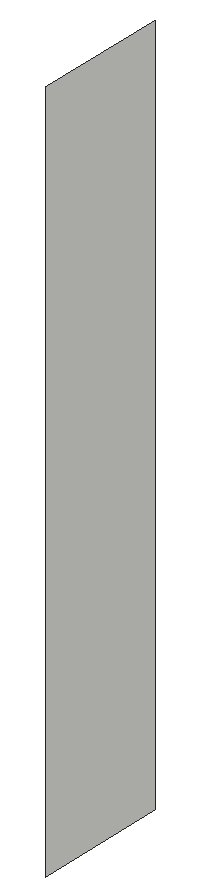
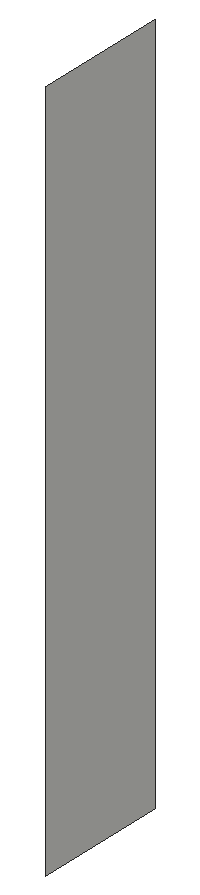
# SketchUp Ruby script. Lengths in inches.
U = 1.inch
M = Sketchup.active_model
def pt(a) = Geom::Point3d.new(a.map { |v| v * U })
def face(e, loops, mat)
  f = e.add_face(loops[0].map { |a| pt(a) })
  loops[1..].each { |l| e.add_face(l.map { |a| pt(a) }).erase! }
  f.material = f.back_material = mat if mat
  f
end
# faces: each face lists its corners as indices into pts; further lists are holes
def faces(e, pts, list, mat = nil) = list.each { |f| face(e, (f[0].is_a?(Array) ? f : [f]).map { |l| l.map { |i| pts[i] } }, mat) }
# xy, xz, yz: faces in a plane at the given z, y or x. An outline is a flat list of corners, or four numbers for a rectangle; further outlines are holes
def ring(l) = l.size == 4 ? [[l[0], l[1]], [l[2], l[1]], [l[2], l[3]], [l[0], l[3]]] : l.each_slice(2).to_a
def flat(e, list, mat, &to3) = list.each { |f| face(e, (f[0].is_a?(Array) ? f : [f]).map { |l| ring(l).map { |u, v| to3.(u, v) } }, mat) }
def xy(e, z, list, mat = nil) = flat(e, list, mat) { |x, y| [x, y, z] }
def xz(e, y, list, mat = nil) = flat(e, list, mat) { |x, z| [x, y, z] }
def yz(e, x, list, mat = nil) = flat(e, list, mat) { |y, z| [x, y, z] }
def lines(e, pts, list) = list.each { |a, b| e.add_line(pt(pts[a]), pt(pts[b])) }
# prism: a flat outline (further loops are holes) pulled along v
def prism(e, loops, v, mat = nil)
  f = face(e, loops, mat); d = Geom::Vector3d.new(v.map { |x| x * U })
  f.pushpull(f.normal.samedirection?(d) ? d.length : -d.length)
end
def box(e, o, s, mat = nil) = prism(e, [[o, [o[0] + s[0], o[1], o[2]], [o[0] + s[0], o[1] + s[1], o[2]], [o[0], o[1] + s[1], o[2]]]], [0, 0, s[2]], mat)
def at(x, y, z, deg = 0) = Geom::Transformation.translation(pt([x, y, z])) * Geom::Transformation.rotation(ORIGIN, Z_AXIS, deg.degrees)
def axes(o, x, y, z) = Geom::Transformation.new([*x, 0, *y, 0, *z, 0, *pt(o).to_a, 1])
def part(name) = M.definitions.add(name)
# library, detail: a bought-in or finely detailed component or shape, given as its bounding box
def library(name, o, s) = part(name).tap { |d| box(d.entities, o, s) }
def detail(e, o, s) = box(e.add_group.entities, o, s)
def put(e, d, t, mat = nil) = e.add_instance(d, t).tap { |i| i.material = mat if mat }
def group(e, t, mat = nil) = e.add_group.tap { |g| g.transformation = t; g.material = mat if mat }.entities
root = M.entities
yz(root,376.86,[[403.76,103.6875,424.53,211.6875]])
